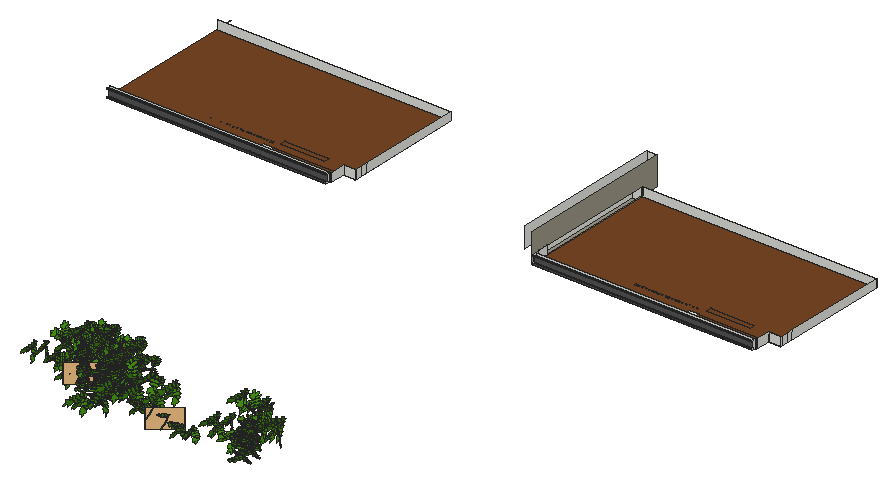
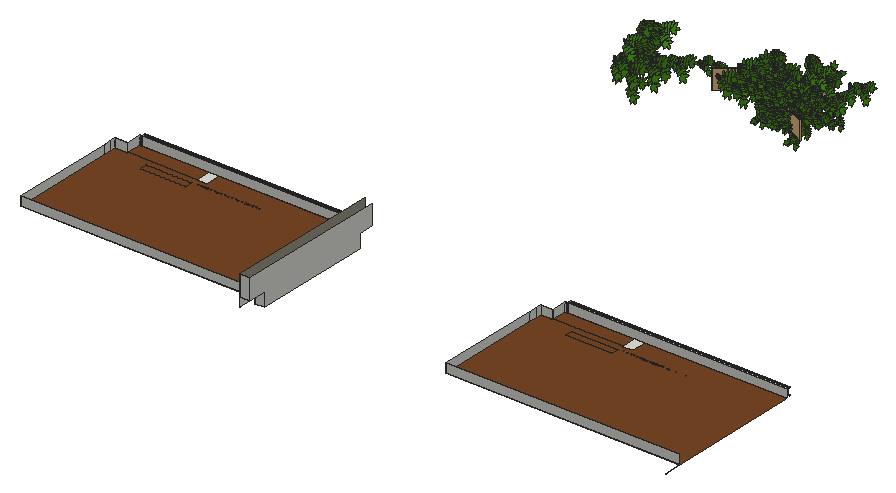
# SketchUp Ruby script. Lengths in inches.
U = 1.inch
M = Sketchup.active_model
def pt(a) = Geom::Point3d.new(a.map { |v| v * U })
def face(e, loops, mat)
  f = e.add_face(loops[0].map { |a| pt(a) })
  loops[1..].each { |l| e.add_face(l.map { |a| pt(a) }).erase! }
  f.material = f.back_material = mat if mat
  f
end
# faces: each face lists its corners as indices into pts; further lists are holes
def faces(e, pts, list, mat = nil) = list.each { |f| face(e, (f[0].is_a?(Array) ? f : [f]).map { |l| l.map { |i| pts[i] } }, mat) }
# xy, xz, yz: faces in a plane at the given z, y or x. An outline is a flat list of corners, or four numbers for a rectangle; further outlines are holes
def ring(l) = l.size == 4 ? [[l[0], l[1]], [l[2], l[1]], [l[2], l[3]], [l[0], l[3]]] : l.each_slice(2).to_a
def flat(e, list, mat, &to3) = list.each { |f| face(e, (f[0].is_a?(Array) ? f : [f]).map { |l| ring(l).map { |u, v| to3.(u, v) } }, mat) }
def xy(e, z, list, mat = nil) = flat(e, list, mat) { |x, y| [x, y, z] }
def xz(e, y, list, mat = nil) = flat(e, list, mat) { |x, z| [x, y, z] }
def yz(e, x, list, mat = nil) = flat(e, list, mat) { |y, z| [x, y, z] }
def lines(e, pts, list) = list.each { |a, b| e.add_line(pt(pts[a]), pt(pts[b])) }
# prism: a flat outline (further loops are holes) pulled along v
def prism(e, loops, v, mat = nil)
  f = face(e, loops, mat); d = Geom::Vector3d.new(v.map { |x| x * U })
  f.pushpull(f.normal.samedirection?(d) ? d.length : -d.length)
end
def box(e, o, s, mat = nil) = prism(e, [[o, [o[0] + s[0], o[1], o[2]], [o[0] + s[0], o[1] + s[1], o[2]], [o[0], o[1] + s[1], o[2]]]], [0, 0, s[2]], mat)
def at(x, y, z, deg = 0) = Geom::Transformation.translation(pt([x, y, z])) * Geom::Transformation.rotation(ORIGIN, Z_AXIS, deg.degrees)
def axes(o, x, y, z) = Geom::Transformation.new([*x, 0, *y, 0, *z, 0, *pt(o).to_a, 1])
def part(name) = M.definitions.add(name)
# library, detail: a bought-in or finely detailed component or shape, given as its bounding box
def library(name, o, s) = part(name).tap { |d| box(d.entities, o, s) }
def detail(e, o, s) = box(e.add_group.entities, o, s)
def put(e, d, t, mat = nil) = e.add_instance(d, t).tap { |i| i.material = mat if mat }
def group(e, t, mat = nil) = e.add_group.tap { |g| g.transformation = t; g.material = mat if mat }.entities
root = M.entities
M.materials.add("[Color M05]").color = [86, 86, 86]
M.materials.add("[Concrete Tile]").color = [155, 150, 134]
M.materials.add("[Wood Veneer 01]").color = [120, 70, 37]
M.materials.add("hojas").color = [70, 150, 19]
c1 = part("rama-acacia")
p = [[-13.53,0.69,-1.07],[-13.38,0.86,-0.98],[-13.61,0.85,-1.06],[-14.07,0.85,-1.21],[-15.17,0.86,-1.58],[-15.95,0.92,-1.83],
  [-16.01,1,-1.83],[-16.01,1.17,-1.78],[-16.07,1.93,-1.6],[-16.4,2.73,-1.5],[-16.65,3.06,-1.5],[-17.13,4.01,-1.41],
  [-17.78,4.7,-1.44],[-18.28,5.07,-1.51],[-18.57,5.18,-1.58],[-18.91,5.47,-1.62],[-19.07,5.48,-1.67],[-19.35,5.61,-1.73],
  [-19.51,5.64,-1.78],[-19.38,5.57,-1.75],[-19.33,5.5,-1.75],[-19.31,5.23,-1.82],[-19.38,5.08,-1.89],[-19.41,4.84,-1.96],
  [-19.36,4.59,-2.01],[-19.43,4.55,-2.04],[-19.36,4.15,-2.125],[-19.21,3.7,-2.19],[-18.875,3.1,-2.24],[-18.61,2.78,-2.24],
  [-17.83,2.19,-2.13],[-17.4375,1.85,-2.09],[-17.04,1.49,-2.05],[-16.61,1.24,-1.97],[-16.17,1.0625,-1.87],[-16.06,0.95,-1.86],
  [-16.06,0.91,-1.87],[-16.32,0.9,-1.96],[-16.7,0.88,-2.1],[-17.05,0.91,-2.21],[-17.61,1.15,-2.33],[-18.06,1.29,-2.45],
  [-18.88,1.53,-2.67],[-20.25,1.46,-3.15],[-20.59,1.49,-3.26],[-20.79,1.37,-3.36],[-21.08,1.2,-3.5],[-21.28,1.22,-3.5625],
  [-21.48,0.94,-3.71],[-21.79,0.5,-3.93],[-22.02,0.17,-4.1],[-22.11,0.05,-4.16],[-22.21,-0.02,-4.21],[-22.375,-0.05,-4.28],
  [-22.375,-0.07,-4.28],[-22.18,-0.09,-4.22],[-22.11,-0.07,-4.19],[-21.78,-0.1,-4.09],[-21.6,-0.18,-4.05],[-21.52,-0.27,-4.04],
  [-21.33,-0.33,-4],[-20.94,-0.54,-3.92],[-20.6875,-0.63,-3.86],[-20.54,-0.68,-3.82],[-20.42,-0.67,-3.78],[-20.09,-0.46,-3.61],
  [-19.8,-0.24,-3.45],[-19.21,-0.02,-3.19],[-18.48,0.08,-2.92],[-17.72,0.38,-2.58],[-17.4,0.5,-2.4375],[-16.93,0.75,-2.21],
  [-16.78,0.8,-2.15],[-16.1,0.83,-1.91],[-16.0625,0.81,-1.9],[-16.08,0.77,-1.91],[-16.27,0.72,-1.99],[-16.88,0.39,-2.29],
  [-17.1875,0.15,-2.46],[-17.27,0.02,-2.52],[-17.94,-0.52,-2.89],[-17.94,-0.59,-2.91],[-18.08,-0.68,-2.99],[-18.13,-0.86,-3.05],
  [-18.56,-1.55,-3.38],[-18.71,-2.11,-3.58],[-18.79,-2.61,-3.74],[-18.86,-2.84,-3.83],[-18.87,-3.07,-3.89],[-18.84,-3.22,-3.92],
  [-18.8,-3.26,-3.92],[-18.76,-3.47,-3.96],[-18.76,-3.6,-4],[-18.67,-3.8,-4.02],[-18.61,-3.92,-4.04],[-18.58,-4.11,-4.07],
  [-18.53,-4.18,-4.08],[-18.58,-4.35,-4.14],[-18.65,-4.43,-4.18],[-18.72,-4.51,-4.23],[-18.8125,-4.51,-4.26],[-18.8125,-4.53,-4.26],
  [-18.72,-4.54,-4.24],[-18.66,-4.49,-4.21],[-18.58,-4.43,-4.16],[-18.35,-4.23,-4.03],[-18.32,-4.17,-4],[-18.22,-4.125,-3.95],
  [-18.1,-4,-3.88],[-17.79,-3.72,-3.7],[-17.68,-3.51,-3.61],[-17.32,-3.13,-3.38],[-17.24,-2.94,-3.31],[-16.78,-2.12,-2.93],
  [-16.48,-1.78,-2.73],[-16.3,-1.28,-2.54],[-16.05,-0.75,-2.3125],[-15.89,-0.2,-2.11],[-15.89,0.39,-1.95],[-15.96,0.79,-1.87],
  [-15.91,0.82,-1.84],[-15.27,0.8,-1.63],[-14.18,0.76,-1.27],[-13.78,0.73,-1.15],[-13.78,0.67,-1.16],[-14.23,0.54,-1.35],
  [-14.65,0.33,-1.55],[-14.97,0.02,-1.74],[-15.25,-0.36,-1.9375],[-15.57,-0.72,-2.14],[-15.96,-1.64,-2.52],[-16.2,-2.51,-2.84],
  [-16.2,-3.12,-3],[-16.14,-3.41,-3.06],[-16.1,-3.75,-3.14],[-16.1,-4.09,-3.23],[-16.2,-4.25,-3.3],[-16.2,-4.28,-3.3125],
  [-16.08,-4.19,-3.24],[-15.98,-4.08,-3.18],[-15.96,-3.94,-3.14],[-15.96,-3.8125,-3.1],[-15.9,-3.72,-3.06],[-15.68,-3.55,-2.9375],
  [-15.51,-3.49,-2.86],[-15.3,-3.33,-2.75],[-15.23,-3.17,-2.68],[-15.01,-3.03,-2.57],[-14.875,-2.83,-2.47],[-14.6,-2.59,-2.3125],
  [-14.4,-2.27,-2.16],[-14.12,-1.6,-1.89],[-13.91,-1.1,-1.68],[-13.67,-0.83,-1.53],[-13.53,-0.45,-1.38],[-13.53,0.67,-1.08],
  [-12.41,6.01,0.65],[-12.44,6.14,0.68],[-12.41,6.29,0.73],[-12.43,6.29,0.73],[-12.44,6.26,0.72],[-12.47,6.15,0.68],
  [-12.49,6.07,0.66],[-12.57,5.75,0.55],[-12.67,5.36,0.43],[-12.79,4.875,0.28],[-12.83,4.52,0.18],[-12.83,3.99,0.04],
  [-12.73,3.11,-0.18],[-12.58,2.52,-0.3125],[-12.3,1.97,-0.41],[-11.88,1.51,-0.46],[-11.37,1.0625,-0.48],[-10.75,0.75,-0.45],
  [-10.75,0.68,-0.47],[-12.55,0.7,-0.79],[-13.21,0.79,-0.89],[-13.2,0.67,-0.92],[-12.56,0.62,-0.82],[-11.15,0.56,-0.58],
  [-10.79,0.54,-0.52],[-10.72,0.52,-0.51],[-10.72,0.5,-0.52],[-10.87,0.47,-0.55],[-11.14,0.41,-0.62],[-11.39,0.27,-0.7],
  [-11.625,-0.01,-0.82],[-11.8,-0.43,-0.96],[-11.83,-0.57,-1],[-12.02,-1.08,-1.17],[-12.1,-1.39,-1.27],[-12.17,-1.95,-1.4375],
  [-12.17,-2.77,-1.65],[-12.09,-3.59,-1.86],[-11.86,-4.26,-2],[-11.8125,-4.4,-2.03],[-11.84,-4.49,-2.05],[-11.91,-4.6,-2.1],
  [-11.97,-4.65,-2.12],[-11.98,-4.67,-2.13],[-11.92,-4.65,-2.11],[-11.84,-4.59,-2.08],[-11.77,-4.52,-2.05],[-11.74,-4.47,-2.03],
  [-11.37,-4.3125,-1.92],[-10.95,-4.0625,-1.78],[-10.82,-3.89,-1.71],[-10.64,-3.57,-1.59],[-10.41,-3.05,-1.41],[-10.27,-2.73,-1.3],
  [-10.07,-1.88,-1.03],[-10.15,-0.71,-0.73],[-10.31,-0.1,-0.6],[-10.5,0.4,-0.5],[-10.5,0.48,-0.48],[-10.44,0.53,-0.45],
  [-10.39,0.64,-0.42],[-10.52,0.73,-0.42],[-10.44,0.93,-0.35],[-10.44,1.2,-0.28],[-10.32,1.47,-0.18],[-10.48,2.6875,0.12],
  [-10.43,2.96,0.2],[-10.75,3.87,0.38],[-11.26,4.93,0.57],[-11.8,5.54,0.64],[-12.37,5.93,0.64],[-7.78,0.19,-0.06],
  [-7.78,0.25,-0.04],[-7.75,0.39,0],[-7.89,0.4,-0.02],[-7.96,0.46,-0.02],[-7.96,0.49,-0.01],[-7.76,0.62,0.06],
  [-7.53,0.99,0.2],[-7.31,1.78,0.45],[-7.31,2.74,0.71],[-7.63,3.6875,0.9],[-8.02,4.57,1.07],[-8.66,5.23,1.13],
  [-8.83,5.4,1.14],[-8.92,5.54,1.16],[-9.1,5.64,1.16],[-9.08,5.6,1.15],[-9.02,5.56,1.15],[-8.94,5.46,1.14],
  [-8.9,5.37,1.12],[-8.9375,5.25,1.08],[-9.14,4.92,0.96],[-9.31,4.5625,0.83],[-9.39,3.73,0.6],[-9.44,2.76,0.32],
  [-9.23,1.59,0.05],[-8.82,0.9,-0.06],[-8.36,0.59,-0.0625],[-8.14,0.51,-0.04],[-8.05,0.48,-0.03],[-8.05,0.46,-0.04],
  [-8.12,0.43,-0.06],[-10.1,0.49,-0.4],[-8.22,0.3125,-0.11],[-8.22,0.25,-0.125],[-8.53,0.13,-0.21],[-8.8,-0.16,-0.34],
  [-8.96,-0.61,-0.49],[-8.96,-0.87,-0.56],[-9.16,-1.42,-0.74],[-9.13,-1.77,-0.83],[-9.09,-1.83,-0.84],[-9.125,-1.92,-0.87],
  [-9.125,-2.13,-0.93],[-9.08,-2.23,-0.95],[-9.15,-2.39,-1],[-9.11,-2.67,-1.07],[-9.03,-2.86,-1.11],[-9.07,-3.03,-1.16],
  [-8.97,-3.23,-1.19],[-8.93,-3.44,-1.24],[-8.93,-3.71,-1.32],[-8.79,-4.05,-1.38],[-8.7,-4.25,-1.42],[-8.7,-4.39,-1.46],
  [-8.76,-4.53,-1.5],[-8.77,-4.65,-1.54],[-8.64,-4.55,-1.49],[-8.27,-4.22,-1.33],[-8.1875,-4.06,-1.27],[-8.07,-3.98,-1.23],
  [-7.98,-3.79,-1.17],[-7.79,-3.59,-1.08],[-7.64,-3.3,-0.97],[-7.64,-3.25,-0.96],[-7.59,-3.21,-0.9375],[-7.52,-2.93,-0.85],
  [-7.52,-2.85,-0.83],[-7.47,-2.81,-0.81],[-7.3,-2.09,-0.59],[-7.32,-2.01,-0.57],[-7.27,-1.95,-0.54],[-7.1875,-1.57,-0.42],
  [-7.17,-1.46,-0.39],[-7.17,-1.16,-0.3125],[-7.23,-0.61,-0.17],[-7.49,-0.15,-0.1],[-13.39,-0.07,-1.23],[-13.39,0.25,-1.14],
  [-13.49,0.5625,-1.09],[-13.8,1.01,-1.08],[-13.61,0.91,-1.04],[-13.38,0.92,-0.96],[-13.32,1.03,-0.91],[-13.32,1.35,-0.82],
  [-13.28,1.49,-0.77],[-13.28,1.99,-0.64],[-13.44,2.67,-0.51],[-13.72,3.31,-0.43],[-13.93,3.71,-0.4],[-14.1,4.39,-0.27],
  [-14.5625,5.06,-0.25],[-14.89,5.62,-0.21],[-15.33,6.1,-0.23],[-15.65,6.8,-0.15],[-15.79,6.89,-0.18],[-15.61,6.52,-0.22],
  [-15.51,6.32,-0.24],[-15.45,6.28,-0.23],[-15.52,6,-0.32],[-15.63,5.6875,-0.45],[-15.77,4.97,-0.68],[-15.7,4.25,-0.85],
  [-15.46,3,-1.11],[-15,2.03,-1.21],[-14.3,1.29,-1.17],[-4.5625,0.33,0.09],[-4.22,0.49,0.13],[-4,0.7,0.1875],
  [-3.86,0.99,0.26],[-3.77,1.41,0.38],[-3.7,1.73,0.46],[-3.77,1.99,0.53],[-3.85,2.17,0.58],[-3.88,2.57,0.6875],
  [-3.98,2.9,0.78],[-4.0625,2.97,0.8],[-4.1,3.14,0.84],[-4.1875,3.25,0.87],[-4.27,3.55,0.95],[-4.31,3.71,0.99],
  [-4.42,3.9,1.04],[-4.625,4.2,1.125],[-4.72,4.39,1.18],[-4.89,4.57,1.23],[-4.98,4.73,1.27],[-5,4.72,1.26],
  [-5.01,4.51,1.21],[-4.96,4.32,1.16],[-4.97,4.27,1.14],[-5.14,3.78,1.01],[-5.3,3.39,0.91],[-5.44,2.76,0.74],
  [-5.5,2.09,0.56],[-5.57,1.78,0.48],[-5.57,1.42,0.38],[-5.57,1.09,0.29],[-5.47,0.72,0.19],[-5.22,0.44,0.12],
  [-4.93,0.27,0.07],[-4.76,0.22,0.06],[-4.76,0.18,0.05],[-4.83,0.16,0.04],[-5.26,0,0],[-5.34,-0.04,-0.01],
  [-5.47,-0.22,-0.06],[-5.51,-0.6,-0.16],[-5.42,-1.09,-0.29],[-5.28,-1.49,-0.4],[-5.21,-1.87,-0.5],[-5.11,-2.15,-0.57],
  [-5.08,-2.34,-0.63],[-5.01,-2.47,-0.66],[-4.96,-2.69,-0.72],[-4.86,-2.9375,-0.79],[-4.84,-3.07,-0.82],[-4.77,-3.18,-0.85],
  [-4.74,-3.43,-0.92],[-4.7,-3.71,-0.99],[-4.62,-3.89,-1.04],[-4.58,-3.98,-1.07],[-4.58,-3.83,-1.03],[-4.51,-3.67,-0.98],
  [-4.3,-3.32,-0.89],[-4.16,-3.09,-0.83],[-4.16,-2.98,-0.8],[-4.11,-2.92,-0.78],[-4.02,-2.8,-0.75],[-3.95,-2.59,-0.69],
  [-3.95,-2.33,-0.625],[-3.86,-2.26,-0.6],[-3.86,-2.02,-0.54],[-3.86,-1.44,-0.39],[-3.94,-1.22,-0.33],[-3.94,-1.08,-0.29],
  [-4,-0.96,-0.26],[-4,-0.87,-0.23],[-4.0625,-0.8125,-0.22],[-4.16,-0.54,-0.14],[-4.39,-0.24,-0.06],[-4.61,-0.08,-0.02],
  [-4.77,-0.03,-0.01],[-4.77,-0.01,0],[-4.65,-0.01,0],[-4.61,0.19,0.05],[-4.66,0.23,0.0625],[-4.63,0.29,0.08],
  [-4.07,0.17,0.04],[0,-0.24,-0.06],[0,0,0],[-0.5,0.04,0.01],[-1.58,0.08,0.02],[-13.78,0.67,-1.08]]
faces(c1.entities,p,[[0,1,2,3,4,5,6,7,8,9,10,11,12,13,14,15,16,17,18,19,20,21,22,23,24,25,26,27,28,29,30,31,32,33,34,35,36,37,38,39,40,41,42,43,44,45,46,47,48,49,50,51,52,53,54,55,56,57,58,59,60,61,62,63,64,65,66,67,68,69,70,71,72,73,74,75,76,77,78,79,80,81,82,83,84,85,86,87,88,89,90,91,92,93,94,95,96,97,98,99,100,101,102,103,104,105,106,107,108,109,110,111,112,113,114,115,116,117,118,119,120,121,122,123,124,125,126,127,128,129,130,131,132,133,134,135,136,137,138,139,140,141,142,143,144,145,146,147,148,149,150,151,152,153,154,155],[156,157,158,159,160,161,162,163,164,165,166,167,168,169,170,171,172,173,174,175,176,177,178,179,180,181,182,183,184,185,186,187,188,189,190,191,192,193,194,195,196,197,198,199,200,201,202,203,204,205,206,207,208,209,210,211,212,213,214,215,216,217,218,219,220,221,222,223,224,225,226],[227,228,229,230,231,232,233,234,235,236,237,238,239,240,241,242,243,244,245,246,247,248,249,250,251,252,253,254,255,256,257,258,216,215,259,260,261,262,263,264,265,266,267,268,269,270,271,272,273,274,275,276,277,278,279,280,281,282,283,284,285,286,287,288,289,290,291,292,293,294,295,296,297,298,299,300,301,302,303],[154,304,305,306,155],[307,308,1,309,310,311,312,313,314,315,316,317,318,319,320,321,322,323,324,325,326,327,328,329,330,331,332],[333,334,335,336,337,338,339,340,341,342,343,344,345,346,347,348,349,350,351,352,353,354,355,356,357,358,359,360,361,362,363,364,365,366,367,368,369,370,371,372,373,374,375,376,377,378,379,380,381,382,383,384,385,386,387,388,389,390,391,392,393,394,395,396,397,398,399,400,401,402,403,404,405,406,407,408,409,410,411,412,413],[0,177,1],[308,2,1],
  [176,1,177],[414,411,410,415,416,417,418],[228,370,229],[369,229,370]],"hojas")
lines(c1.entities,p,[[155,419]])
c2 = part("Group\#150")
put(c2.entities,c1,axes([10.13,10.27,0],[0.45315,0.21131,0],[-0.21131,0.45315,0],[0,0,0.5]))
put(c2.entities,c1,axes([10.13,10.27,0],[0.11638,0.47539,0.10227],[-0.48087,0.12813,-0.0484],[-0.07223,-0.08709,0.48703]))
put(c2.entities,c1,axes([9.58,10.26,-0.7],[0.1449,0.38901,-0.2787],[-0.10883,0.31035,0.37662],[0.46601,-0.04848,0.17461]))
c3 = part("Group\#151")
put(c3.entities,c2,axes([24.99,4.24,9.59],[0.78856,0.61496,0],[0.01473,-0.01889,0.99971],[0.61478,-0.78833,-0.02396]))
put(c3.entities,c2,axes([39.5,6.625,12.55],[0.6544,0.49291,0.57341],[-0.44023,-0.3682,0.81892],[0.61478,-0.78833,-0.02396]))
put(c3.entities,c2,axes([32.34,3.7,6.88],[0.78856,0.61496,0],[0.01473,-0.01889,0.99971],[0.61478,-0.78833,-0.02396]))
put(c3.entities,c2,axes([43.14,6.65,17.54],[0.78856,0.61496,0],[0.35273,-0.4523,0.81915],[0.50374,-0.64595,-0.57358]))
put(c3.entities,c2,axes([12.2,6.2,16.68],[0.7209,0.54936,0.4225],[-0.31991,-0.27701,0.90605],[0.61478,-0.78833,-0.02396]))
put(c3.entities,c2,axes([49.9375,3.79,26.09],[0.78856,0.61496,0],[0.01473,-0.01889,0.99971],[0.61478,-0.78833,-0.02396]))
put(c3.entities,c2,axes([36.11,4.9375,33.94],[0.78856,0.61496,0],[0.01473,-0.01889,0.99971],[0.61478,-0.78833,-0.02396]))
put(c3.entities,c2,axes([39.61,3.79,23.47],[0.78856,0.61496,0],[0.01473,-0.01889,0.99971],[0.61478,-0.78833,-0.02396]))
put(c3.entities,c2,axes([25.59,6.5625,46.47],[-0.40704,-0.29112,-0.86578],[0.67555,0.54201,-0.49986],[0.61478,-0.78833,-0.02396]))
put(c3.entities,c2,axes([54.97,1.98,11.65],[0.78856,0.61496,0],[0.01473,-0.01889,0.99971],[0.61478,-0.78833,-0.02396]))
put(c3.entities,c2,axes([32.97,3.79,19.14],[0.78856,0.61496,0],[0.01473,-0.01889,0.99971],[0.61478,-0.78833,-0.02396]))
put(c3.entities,c2,axes([24.24,3.79,21.99],[0.78856,0.61496,0],[0.01473,-0.01889,0.99971],[0.61478,-0.78833,-0.02396]))
put(c3.entities,c2,axes([16.86,4.24,12.3],[0.78856,0.61496,0],[0.01473,-0.01889,0.99971],[0.61478,-0.78833,-0.02396]))
put(c3.entities,c2,axes([1.23,3.9375,19.07],[0.78856,0.61496,0],[0.01473,-0.01889,0.99971],[0.61478,-0.78833,-0.02396]))
put(c3.entities,c2,axes([29.05,5.25,29.11],[0.78856,0.61496,0],[0.21033,-0.2697,0.93969],[0.57787,-0.741,-0.34202]))
put(c3.entities,c2,axes([24.16,3.79,-0.1],[0.78856,0.61496,0],[0.01473,-0.01889,0.99971],[0.61478,-0.78833,-0.02396]))
c4 = library("Group\#152",[0,0,0],[130.24,0.88,39.6])
xy(root,254.125,[[2992.01,877.14,2992.01,1122.97,3012.13,1122.97,3012.76,877.14]],"[Concrete Tile]")
xy(root,264.75,[[2427.73,840.97,2447.38,845.35],[3307.68,840.97,3327.33,845.35],[2427.73,845.35,2447.38,877.14],[2587.8,845.35,2591.89,846.1],[3307.68,845.35,3327.33,877.14],
  [3467.75,845.35,3471.83,846.1],[2591.89,877.14,2617.01,877.51],[3471.83,877.14,3496.96,877.51]])
xy(root,264.75,[[2427.73,837.03,2447.38,840.97],[2447.38,837.03,2587.8,845.35],[3014.7,837.03,3307.68,845.35],[3307.68,837.03,3327.33,840.97],[3327.33,837.03,3467.75,845.35],
  [[2134.75,845.35,2134.75,850.97,2132.8125,850.97,2132.8125,877.14,2132.1875,1122.97,2132.1875,1160.85,2132.8125,1160.85,2132.8125,1122.97,2617.01,1122.97,2617.01,877.51,2591.89,877.51,2591.89,877.14,2427.73,877.14,2427.73,845.35],[2447.58,890.39,2542.64,905.7],[2410.11,888.83,2415.52,890.39],[2424.11,888.83,2429.52,890.39],[2417.11,888.83,2422.52,890.39],[2431.11,888.83,2436.52,890.39],[2403.11,888.83,2408.52,890.39],[2396.11,888.83,2401.52,890.39],[2305.05,888.95,2310.46,890.39],[2340.11,888.95,2345.52,890.39],[2361.11,888.95,2366.52,890.39],[2312.11,888.95,2317.52,890.39],[2389.11,888.95,2394.52,890.39],[2382.11,888.95,2387.52,890.39],[2368.11,888.95,2373.52,890.39],[2375.11,888.95,2380.52,890.39],[2319.11,888.95,2324.52,890.39],[2333.11,888.95,2338.52,890.39],[2347.11,888.95,2352.52,890.39],[2354.11,888.95,2359.52,890.39],[2326.11,888.95,2331.52,890.39]],[2447.38,845.35,2447.38,877.14,2591.89,877.14,2591.89,846.1,2587.8,846.1,2587.8,845.35],[[3014.7,845.35,3014.7,850.97,3012.76,850.97,3012.76,877.14,3012.13,1122.97,3012.13,1160.85,3012.76,1160.85,3012.76,1122.97,3496.96,1122.97,3496.96,877.51,3471.83,877.51,3471.83,877.14,3307.68,877.14,3307.68,845.35],[3327.52,890.39,3422.58,905.7],[3290.05,888.83,3295.47,890.39],[3304.05,888.83,3309.47,890.39],[3297.05,888.83,3302.47,890.39],[3311.05,888.83,3316.47,890.39],[3283.05,888.83,3288.47,890.39],[3276.05,888.83,3281.47,890.39],[3184.99,888.95,3190.41,890.39],[3220.05,888.95,3225.47,890.39],[3241.05,888.95,3246.47,890.39],[3192.05,888.95,3197.47,890.39],[3269.05,888.95,3274.47,890.39],[3262.05,888.95,3267.47,890.39],[3248.05,888.95,3253.47,890.39],[3255.05,888.95,3260.47,890.39],[3199.05,888.95,3204.47,890.39],[3213.05,888.95,3218.47,890.39],[3227.05,888.95,3232.47,890.39],[3234.05,888.95,3239.47,890.39],[3206.05,888.95,3211.47,890.39]],[3327.33,845.35,3327.33,877.14,3471.83,877.14,3471.83,846.1,3467.75,846.1,3467.75,845.35],[2396.11,888.83,2401.52,890.39],
  [2403.11,888.83,2408.52,890.39],[2410.11,888.83,2415.52,890.39],[2417.11,888.83,2422.52,890.39],[2424.11,888.83,2429.52,890.39],[2431.11,888.83,2436.52,890.39],
  [3276.05,888.83,3281.47,890.39],[3283.05,888.83,3288.47,890.39],[3290.05,888.83,3295.47,890.39],[3297.05,888.83,3302.47,890.39],[3304.05,888.83,3309.47,890.39],
  [3311.05,888.83,3316.47,890.39],[2340.11,888.95,2345.52,890.39],[2347.11,888.95,2352.52,890.39],[2354.11,888.95,2359.52,890.39],[2361.11,888.95,2366.52,890.39],
  [2368.11,888.95,2373.52,890.39],[2375.11,888.95,2380.52,890.39],[2382.11,888.95,2387.52,890.39],[2389.11,888.95,2394.52,890.39],[3184.99,888.95,3190.41,890.39],
  [3192.05,888.95,3197.47,890.39],[3199.05,888.95,3204.47,890.39],[3206.05,888.95,3211.47,890.39],[3213.05,888.95,3218.47,890.39],[3220.05,888.95,3225.47,890.39],
  [3227.05,888.95,3232.47,890.39],[3234.05,888.95,3239.47,890.39],[3241.05,888.95,3246.47,890.39],[3248.05,888.95,3253.47,890.39],[3255.05,888.95,3260.47,890.39],
  [3262.05,888.95,3267.47,890.39],[3269.05,888.95,3274.47,890.39],[2447.58,890.39,2542.64,905.7],[3327.52,890.39,3422.58,905.7]],"[Wood Veneer 01]")
xy(root,266.9375,[[2427.73,837.03,2447.38,840.97],[2447.38,837.03,2587.8,840.97],[3014.7,837.03,3307.68,840.97],[3307.68,837.03,3327.33,840.97],[3327.33,837.03,3467.75,840.97]])
xy(root,280.5625,[[2134.75,837.03,2587.8,840.97],[3014.7,837.03,3467.75,840.97]])
xz(root,837.03,[[2134.75,264.75,2587.8,266.9375],[3014.7,264.75,3467.75,266.9375],[2134.75,280.5625,2587.8,282.75],[3014.7,280.5625,3467.75,282.75]],"[Color M05]")
xz(root,840.97,[[2134.75,266.9375,2587.8,280.5625],[3014.7,266.9375,3467.75,280.5625]],"[Color M05]")
xz(root,845.35,[[2134.75,264.75,2587.8,282.75],[2587.8,264.75,2591.89,282.75],[3014.7,264.75,3467.75,282.75],[3467.75,264.75,3471.83,282.75]])
xz(root,850.97,[[3012.76,264.75,3014.7,282.75]])
xz(root,877.14,[[2992.01,254.125,3012.76,282.75],[2591.89,264.75,2617.01,282.75],[3471.83,264.75,3496.96,282.75]])
xz(root,877.51,[[2591.89,264.75,2617.01,282.75],[3471.83,264.75,3496.96,282.75]])
xz(root,1122.97,[[2992.01,254.125,3012.13,282.75],[2134.75,264.75,2617.01,282.75],[3012.76,264.75,3014.7,282.75],[3014.7,264.75,3496.96,282.75]])
xz(root,1160.85,[[3012.13,264.75,3012.13,282.75,2992.01,282.75,2992.01,324.5625,3012.76,324.5625,3012.76,264.75]])
yz(root,2587.8,[[837.03,264.75,840.97,266.9375],[840.97,264.75,845.35,282.75],[837.03,280.5625,840.97,282.75]])
yz(root,2591.89,[[845.35,264.75,846.1,282.75],[846.1,264.75,877.14,282.75],[877.14,264.75,877.51,282.75]])
yz(root,2617.01,[[877.14,264.75,877.51,282.75],[877.51,264.75,890.39,282.75],[890.39,264.75,905.7,282.75],[905.7,264.75,1122.97,282.75]])
yz(root,2992.01,[[877.14,254.125,877.14,282.75,845.35,282.75,845.35,324.5625,1160.85,324.5625,1160.85,282.75,1122.97,282.75,1122.97,254.125]])
yz(root,3012.13,[[1122.97,264.75,1160.85,282.75]])
yz(root,3012.76,[[845.35,264.75,850.97,282.75],[850.97,264.75,877.14,282.75]])
yz(root,3012.76,[[837.03,264.75,845.35,264.75,845.35,282.75,1122.97,282.75,1122.97,264.75,1160.85,264.75,1160.85,324.5625,837.03,324.5625]],"[Concrete Tile]")
yz(root,3014.7,[[837.03,264.75,837.03,266.9375,840.97,266.9375,840.97,280.5625,837.03,280.5625,837.03,282.75,845.35,282.75,845.35,264.75],[845.35,264.75,850.97,282.75]])
yz(root,3467.75,[[837.03,264.75,840.97,266.9375],[840.97,264.75,845.35,282.75],[837.03,280.5625,840.97,282.75]])
yz(root,3471.83,[[845.35,264.75,846.1,282.75],[846.1,264.75,877.14,282.75],[877.14,264.75,877.51,282.75]])
yz(root,3496.96,[[877.14,264.75,877.51,282.75],[877.51,264.75,890.39,282.75],[890.39,264.75,905.7,282.75],[905.7,264.75,1122.97,282.75]])
p = [[3012.13,1122.97,264.75],[3012.76,877.14,264.75],[3012.76,877.14,254.125],[3012.13,1122.97,254.125]]
faces(root,p,[[0,1,2,3]],"[Concrete Tile]")
put(root,c3,axes([2707.375,218.63,232.41],[-1.52983,-1.82319,0],[1.82319,-1.52983,0],[0,0,2.38]))
put(root,c3,axes([2620.08,3.7,252.63],[1.99873,1.39953,0],[-2.79905,3.99746,0],[0,0,2.44]))
put(root,c3,axes([2608.64,128.88,246.21],[2.21,0,0],[0,2.21,0],[0,0,2.21]))
put(root,c4,axes([2669.98,55.21,265.83],[0.39163,0.31085,0],[-0.12434,0.15665,0],[0,0,1]))
put(root,c3,axes([2645.8,110.56,261.77],[1.28558,-1.53209,0],[1.53209,1.28558,0],[0,0,2]))
put(root,c3,at(2668.62,89.75,248.9))
put(root,c4,at(2646.37,169.99,265.26,-26.56))
put(root,c3,axes([2660.02,174.75,252.05],[0.905,-1.56751,0],[2.89989,1.67425,0],[0,0,1.81]))
put(root,c3,axes([2669.36,131.99,230.89],[0.905,-1.56751,0],[2.89989,1.67425,0],[0,0,1.81]))
put(root,c3,axes([2669.36,134.07,230.89],[0.905,-1.56751,0],[2.89989,1.67425,0],[0,0,1.81]))
put(root,c2,axes([2721.01,-0.9,242.49],[0.80931,3.79087,0],[0.09082,-0.01939,3.87519],[3.78978,-0.80908,-0.09287]))
put(root,c3,axes([2673.89,114.18,246.21],[2.21,0,0],[0,2.21,0],[0,0,2.21]))
put(root,c3,at(2717.51,99.64,237.96))
put(root,c3,axes([2704.84,141.04,261.77],[1.14715,-1.6383,0],[1.6383,1.14715,0],[0,0,2]))
put(root,c2,axes([2747.95,33.15,233.23],[0.77187,3.4275,1.63772],[-0.25972,-1.61966,3.51211],[3.78978,-0.80908,-0.09287]))
put(root,c2,axes([2762.1,29.11,268.96],[0.80931,3.79087,0],[0.09082,-0.01939,3.87519],[3.78978,-0.80908,-0.09287]))
put(root,c2,axes([2786.81,67.59,348.73],[-0.48331,-1.87864,-3.35601],[0.65548,3.29269,-1.93759],[3.78978,-0.80908,-0.09287]))
put(root,c2,axes([2789.7,55.99,253.82],[0.80931,3.79087,0],[0.09082,-0.01939,3.87519],[3.78978,-0.80908,-0.09287]))
put(root,c2,axes([2800.33,72.29,281.42],[0.80931,3.79087,0],[1.29655,-0.2768,3.64253],[3.56225,-0.76051,-1.32577]))
put(root,c2,axes([2815.62,77.73,242.77],[0.80931,3.79087,0],[0.09082,-0.01939,3.87519],[3.78978,-0.80908,-0.09287]))
put(root,c2,axes([2814.27,43.53,269.57],[2.49644,0.12893,-0.03435],[0.03683,-0.04723,2.49928],[0.12825,-2.49623,-0.04906]))
put(root,c2,axes([2831.86,49.15,262.12],[1.9714,1.53739,0],[0.03683,-0.04723,2.49928],[1.53695,-1.97083,-0.05989]))
put(root,c2,axes([2835.33,94.28,259.54],[0.80931,3.79087,0],[0.09082,-0.01939,3.87519],[3.78978,-0.80908,-0.09287]))
put(root,c4,axes([2839.02,54.57,241.81],[0.39163,0.31085,0],[-0.12434,0.15665,0],[0,0,1]))
put(root,c2,axes([2850.7,63.95,243.67],[1.9714,1.53739,0],[0.03683,-0.04723,2.49928],[1.53695,-1.97083,-0.05989]))
put(root,c2,axes([2883.28,56.76,244.24],[2.57212,0.59147,-0.06301],[0.06264,0.00875,2.63924],[0.59151,-2.57288,-0.00551]))
put(root,c2,axes([2930.09,45.38,243.99],[-0.36508,2.61463,0],[0.06264,0.00875,2.63924],[2.61388,0.36498,-0.06325]))
put(root,c2,axes([2938.69,74.37,251.62],[0.37045,4.09667,0],[0.08998,-0.06733,3.00354],[3.7549,-2.80958,-0.07198]))
put(root,c2,axes([2949.2,133.1875,272.72],[0.37045,4.09667,0],[0.08998,-0.06733,3.00354],[3.7549,-2.80958,-0.07198]))
put(root,c2,axes([2957.05,78.125,243.99],[-0.36508,2.61463,0],[0.06264,0.00875,2.63924],[2.61388,0.36498,-0.06325]))
put(root,c2,axes([2961.04,101.5625,244.44],[0.37377,3.68439,1.26935],[-0.07501,-1.79235,2.72213],[3.7549,-2.80958,-0.07198]))
put(root,c2,axes([2977.7,154.1875,233.93],[0.37045,4.09667,0],[0.08998,-0.06733,3.00354],[3.7549,-2.80958,-0.07198]))
put(root,c2,axes([2977.7,154.1875,259.1],[0.37045,4.09667,0],[0.08998,-0.06733,3.00354],[3.7549,-2.80958,-0.07198]))
put(root,c2,axes([2978.51,99.28,231.28],[0.37045,4.09667,0],[0.08998,-0.06733,3.00354],[3.7549,-2.80958,-0.07198]))
put(root,c2,axes([2994.89,123.4,333.96],[-0.26315,-1.99002,-2.60114],[0.27583,3.58148,-1.50177],[3.7549,-2.80958,-0.07198]))
put(root,c2,axes([2998.96,108.23,260.4],[0.37045,4.09667,0],[0.08998,-0.06733,3.00354],[3.7549,-2.80958,-0.07198]))
put(root,c3,axes([2969.89,131.99,230.89],[0.905,-1.56751,0],[2.89989,1.67425,0],[0,0,1.81]))
put(root,c2,axes([2998.47,39.29,269.66],[0.37045,4.09667,0],[2.15434,-1.61197,2.46106],[3.07672,-2.30213,-1.72325]))
put(root,c2,axes([3007.47,122.36,281.79],[0.37045,4.09667,0],[1.28462,-0.96121,2.82321],[3.52946,-2.6409,-1.02757]))
put(root,c2,axes([3021.66,121.34,251.84],[0.37045,4.09667,0],[0.08998,-0.06733,3.00354],[3.7549,-2.80958,-0.07198]))
put(root,c2,axes([3026.69,131.5,248.42],[0.37045,4.09667,0],[0.08998,-0.06733,3.00354],[3.7549,-2.80958,-0.07198]))
put(root,c2,axes([3030.9,144.59,232.05],[0.35507,3.31717,1.72276],[-0.13877,-2.4049,2.46035],[3.7549,-2.80958,-0.07198]))
put(root,c2,axes([3030.18,85.14,264.84],[0.37045,4.09667,0],[0.08998,-0.06733,3.00354],[3.7549,-2.80958,-0.07198]))
